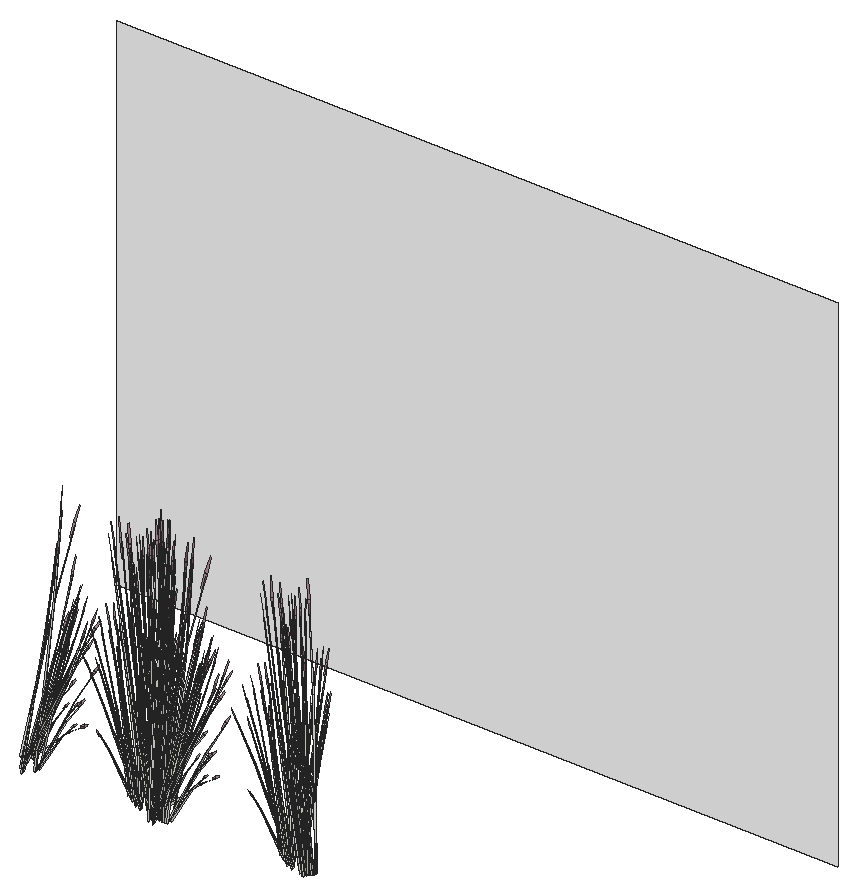
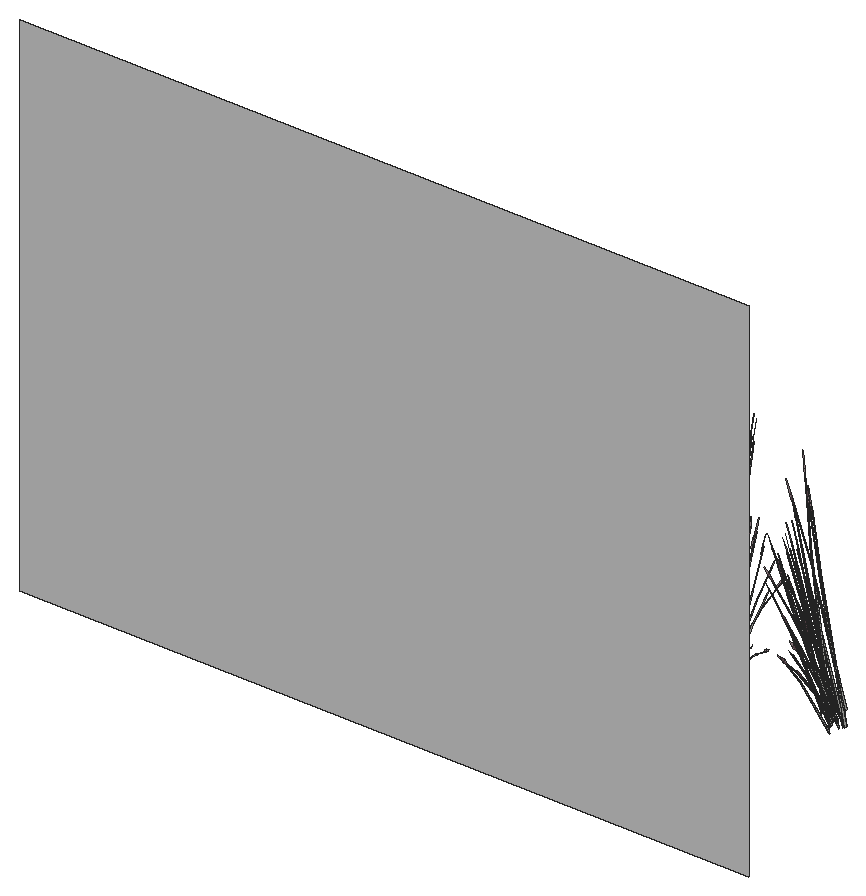
# SketchUp Ruby script. Lengths in inches.
U = 1.inch
M = Sketchup.active_model
def pt(a) = Geom::Point3d.new(a.map { |v| v * U })
def face(e, loops, mat)
  f = e.add_face(loops[0].map { |a| pt(a) })
  loops[1..].each { |l| e.add_face(l.map { |a| pt(a) }).erase! }
  f.material = f.back_material = mat if mat
  f
end
# faces: each face lists its corners as indices into pts; further lists are holes
def faces(e, pts, list, mat = nil) = list.each { |f| face(e, (f[0].is_a?(Array) ? f : [f]).map { |l| l.map { |i| pts[i] } }, mat) }
# xy, xz, yz: faces in a plane at the given z, y or x. An outline is a flat list of corners, or four numbers for a rectangle; further outlines are holes
def ring(l) = l.size == 4 ? [[l[0], l[1]], [l[2], l[1]], [l[2], l[3]], [l[0], l[3]]] : l.each_slice(2).to_a
def flat(e, list, mat, &to3) = list.each { |f| face(e, (f[0].is_a?(Array) ? f : [f]).map { |l| ring(l).map { |u, v| to3.(u, v) } }, mat) }
def xy(e, z, list, mat = nil) = flat(e, list, mat) { |x, y| [x, y, z] }
def xz(e, y, list, mat = nil) = flat(e, list, mat) { |x, z| [x, y, z] }
def yz(e, x, list, mat = nil) = flat(e, list, mat) { |y, z| [x, y, z] }
def lines(e, pts, list) = list.each { |a, b| e.add_line(pt(pts[a]), pt(pts[b])) }
# prism: a flat outline (further loops are holes) pulled along v
def prism(e, loops, v, mat = nil)
  f = face(e, loops, mat); d = Geom::Vector3d.new(v.map { |x| x * U })
  f.pushpull(f.normal.samedirection?(d) ? d.length : -d.length)
end
def box(e, o, s, mat = nil) = prism(e, [[o, [o[0] + s[0], o[1], o[2]], [o[0] + s[0], o[1] + s[1], o[2]], [o[0], o[1] + s[1], o[2]]]], [0, 0, s[2]], mat)
def at(x, y, z, deg = 0) = Geom::Transformation.translation(pt([x, y, z])) * Geom::Transformation.rotation(ORIGIN, Z_AXIS, deg.degrees)
def axes(o, x, y, z) = Geom::Transformation.new([*x, 0, *y, 0, *z, 0, *pt(o).to_a, 1])
def part(name) = M.definitions.add(name)
# library, detail: a bought-in or finely detailed component or shape, given as its bounding box
def library(name, o, s) = part(name).tap { |d| box(d.entities, o, s) }
def detail(e, o, s) = box(e.add_group.entities, o, s)
def put(e, d, t, mat = nil) = e.add_instance(d, t).tap { |i| i.material = mat if mat }
def group(e, t, mat = nil) = e.add_group.tap { |g| g.transformation = t; g.material = mat if mat }.entities
root = M.entities
M.materials.add("LightPink_Translucent").color = [144, 107, 117]
M.materials["LightPink_Translucent"].alpha = 0.75
M.materials.add("M00_Soft_Cloud").color = [255, 255, 255]
c1 = part("blade")
p = [[2.15,0.21,22],[0,0.17,0],[0.09,0.45,0],[2.18,0.31,22],[2.29,0.31,22],[0.38,0.45,0],
  [2.48,0.24,33],[2.49,0.24,33],[2.48,0.22,33]]
faces(c1.entities,p,[[0,1,2,3],[4,5,2,3],[6,3,4,7],[8,0,3,6]])
c2 = part("seeds")
p = [[0.3,-0.1,1.38],[-0.01,-0.03,1.59],[-0.01,-0.03,0.03],[0.14,-0.07,-0.07],[0.29,-0.03,3],[0.15,0.01,3.11]]
faces(c2.entities,p,[[0,1,2,3],[1,0,4,5]],"LightPink_Translucent")
c3 = part("blade with seeds")
put(c3.entities,c1,at(0,0,0))
put(c3.entities,c2,axes([2.4,0.25,30.99],[1.5799,-0.05474,1.17369],[-0.12525,1.92788,0.29478],[-0.07173,-0.02425,1.56792]))
xz(root,72.98,[[57,0,228,120]],"M00_Soft_Cloud")
put(root,c3,axes([113.61,13.07,-3.79],[0.85008,0,0],[0,0.63259,0],[0,0,1.78407]))
put(root,c3,axes([112.17,13.87,-3.33],[-0.76714,0.40567,-0.29095],[-0.51013,-0.57321,-0.50002],[-0.18927,-0.05821,1.59708]))
put(root,c3,axes([148.18,13.87,-3.33],[-0.76714,0.40567,-0.29095],[-0.51013,-0.57321,-0.50002],[-0.18927,-0.05821,1.59708]))
put(root,c3,axes([113.85,11.59,-3.53],[-0.81646,0.16218,0.17642],[-0.20161,-0.60355,0.35086],[0.07282,0.08794,1.60407]))
put(root,c3,axes([83.18,12.86,-2.125],[-0.31515,0.01384,1.71376],[0.20907,-0.5998,0.13857],[0.44912,0.0371,0.73262]))
put(root,c3,axes([114.35,12.86,-2.125],[-0.31515,0.01384,1.71376],[0.20907,-0.5998,0.13857],[0.44912,0.0371,0.73262]))
put(root,c3,axes([83.59,11.56,-3.97],[0.17848,0.53243,-0.30978],[-0.70886,0.15119,0.30978],[0.1429,0.0614,1.38974]))
put(root,c3,axes([114.76,11.56,-3.97],[0.17848,0.53243,-0.30978],[-0.70886,0.15119,0.30978],[0.1429,0.0614,1.38974]))
put(root,c3,axes([84.81,13.6875,-1.27],[0.27906,0.41663,0.0643],[-0.50888,0.20393,0.50621],[0.22432,-0.04024,0.77189]))
put(root,c3,axes([115.98,13.6875,-1.27],[0.27906,0.41663,0.0643],[-0.50888,0.20393,0.50621],[0.22432,-0.04024,0.77189]))
put(root,c3,axes([113.34,12.75,-3.62],[-0.96033,-0.12874,0.49198],[0.19544,-0.7271,0.19306],[0.14034,0.07021,1.70813]))
put(root,c3,axes([84.75,13.54,-1.27],[-0.21466,0.55714,0.48003],[-0.70573,-0.19051,0.3958],[0.27753,-0.03348,0.9933]))
put(root,c3,axes([115.93,13.54,-1.27],[-0.21466,0.55714,0.48003],[-0.70573,-0.19051,0.3958],[0.27753,-0.03348,0.9933]))
put(root,c3,axes([112.57,14.55,-3.8],[-0.24791,-0.5268,0],[0.70791,-0.18448,0],[0,0,1.54371]))
put(root,c3,axes([112.1,14.05,-3.38],[-0.14658,0.54532,0.1448],[-0.71613,-0.09466,-0.41347],[-0.13033,-0.05599,1.26744]))
put(root,c3,axes([148.11,14.05,-3.38],[-0.14658,0.54532,0.1448],[-0.71613,-0.09466,-0.41347],[-0.13033,-0.05599,1.26744]))
put(root,c3,axes([109.32,12.63,-0.95],[0.63144,0.17046,0.35414],[-0.18417,0.49731,-0.4572],[-0.25423,0.0456,0.87481]))
put(root,c3,axes([145.33,12.63,-0.95],[0.63144,0.17046,0.35414],[-0.18417,0.49731,-0.4572],[-0.25423,0.0456,0.87481]))
put(root,c3,axes([113.5,14.47,-3.82],[0.79769,-0.20732,-0.19198],[0.2803,0.59721,0.00008],[0.08805,-0.02292,1.73897]))
put(root,c3,axes([113.77,14.72,-3.53],[0.21949,-0.60727,0.17642],[0.8032,0.17185,0.35086],[-0.13875,0.00296,1.60407]))
put(root,c3,axes([149.79,14.72,-3.53],[0.21949,-0.60727,0.17642],[0.8032,0.17185,0.35086],[-0.13875,0.00296,1.60407]))
put(root,c3,axes([113.59,13.34,-3.79],[0.53038,0.39469,0],[-0.53038,0.39469,0],[0,0,1.69266]))
put(root,c3,axes([110.58,12.6,-2.66],[0.21597,-0.08839,1.77064],[0.07448,0.61717,0.13857],[-0.4678,0.08189,0.63284]))
put(root,c3,axes([146.59,12.6,-2.66],[0.21597,-0.08839,1.77064],[0.07448,0.61717,0.13857],[-0.4678,0.08189,0.63284]))
put(root,c3,axes([115.03,13.17,-3.53],[-0.59697,-0.44509,0.17642],[0.60159,-0.4317,0.35086],[-0.06593,0.0909,1.60407]))
put(root,c3,axes([82.75,12.5,-3.94],[0.79037,0.10018,-0.62353],[-0.16679,0.61794,-0.16365],[0.23587,0.07488,1.37633]))
put(root,c3,axes([113.92,12.5,-3.94],[0.79037,0.10018,-0.62353],[-0.16679,0.61794,-0.16365],[0.23587,0.07488,1.37633]))
put(root,c3,axes([86.24,13.58,-3.23],[-0.46945,0.10088,1.1486],[0.22097,-0.4169,0.84392],[0.24904,0.02853,0.25299]))
put(root,c3,axes([117.41,13.58,-3.23],[-0.46945,0.10088,1.1486],[0.22097,-0.4169,0.84392],[0.24904,0.02853,0.25299]))
put(root,c3,axes([112.39,14.78,-3.8],[-0.76598,-0.27433,0],[0.36864,-0.57001,0],[0,0,1.62707]))
put(root,c3,axes([148.41,14.78,-3.8],[-0.76598,-0.27433,0],[0.36864,-0.57001,0],[0,0,1.62707]))
put(root,c3,axes([113.03,14.05,-3.54],[-0.74193,-0.49181,-0.25192],[0.6243,-0.55226,0.5513],[-0.19979,0.05753,1.68216]))
put(root,c3,axes([149.04,14.05,-3.54],[-0.74193,-0.49181,-0.25192],[0.6243,-0.55226,0.5513],[-0.19979,0.05753,1.68216]))
put(root,c3,axes([111.08,15,-3.52],[0.7111,0.30552,0.49651],[-0.42504,0.54784,0],[-0.16196,-0.06958,1.57504]))
put(root,c3,axes([147.09,15,-3.52],[0.7111,0.30552,0.49651],[-0.42504,0.54784,0],[-0.16196,-0.06958,1.57504]))
put(root,c3,axes([113.58,12.88,-3.28],[0.36864,-0.55059,0.44739],[0.76598,0.26498,-0.21531],[0,0.12692,1.43643]))
put(root,c3,axes([86.02,15.34,-1.29],[-0.0687,-0.05349,1.77383],[0.15029,-0.57341,-0.16761],[0.27062,-0.03664,0.31391]))
put(root,c3,axes([117.2,15.34,-1.29],[-0.0687,-0.05349,1.77383],[0.15029,-0.57341,-0.16761],[0.27062,-0.03664,0.31391]))
put(root,c3,axes([108.25,13.02,-1.28],[-0.12407,0.07933,1.74944],[0.01055,0.57963,-0.27667],[-0.2844,0.07538,0.14031]))
put(root,c3,axes([144.27,13.02,-1.28],[-0.12407,0.07933,1.74944],[0.01055,0.57963,-0.27667],[-0.2844,0.07538,0.14031]))
put(root,c3,axes([113.44,13.2,-3.71],[0,0.70667,-0.05637],[-0.95008,0,0],[0,0.02221,1.79368]))
put(root,c3,axes([109.09,12.94,-1.32],[-0.20584,0.55581,-0.51099],[-0.70573,-0.19051,-0.3958],[-0.28414,0.05097,0.97773]))
put(root,c3,axes([145.1,12.94,-1.32],[-0.20584,0.55581,-0.51099],[-0.70573,-0.19051,-0.3958],[-0.28414,0.05097,0.97773]))
put(root,c3,axes([109.05,12.46,-0.97],[0.38229,0.5533,-0.1216],[-0.6785,0.2719,-0.67495],[-0.28593,0.073,1.02557]))
put(root,c3,axes([145.07,12.46,-0.97],[0.38229,0.5533,-0.1216],[-0.6785,0.2719,-0.67495],[-0.28593,0.073,1.02557]))
put(root,c3,axes([82.34,12.7,-3.79],[0.45644,0.51287,-0.44739],[-0.69137,0.36116,0.21531],[0.14771,0.06346,1.43643]))
put(root,c3,axes([113.51,12.7,-3.79],[0.45644,0.51287,-0.44739],[-0.69137,0.36116,0.21531],[0.14771,0.06346,1.43643]))
put(root,c3,axes([85.42,14.87,-2.07],[-0.14542,-0.51365,-0.03492],[0.68734,-0.11809,-0.15832],[0.14353,0.03256,0.52218]))
put(root,c3,axes([116.6,14.87,-2.07],[-0.14542,-0.51365,-0.03492],[0.68734,-0.11809,-0.15832],[0.14353,0.03256,0.52218]))
put(root,c3,axes([110.67,15.32,-3.625],[-0.47504,0.61229,0],[-0.79476,-0.34146,-0.51607],[-0.18101,-0.07777,1.63711]))
put(root,c3,axes([146.68,15.32,-3.625],[-0.47504,0.61229,0],[-0.79476,-0.34146,-0.51607],[-0.18101,-0.07777,1.63711]))
put(root,c3,axes([83.64,14.85,-0.97],[0.04068,-0.62141,-0.1216],[0.77029,0.01698,-0.67495],[0.29667,0.04317,1.02557]))
put(root,c3,axes([114.82,14.85,-0.97],[0.04068,-0.62141,-0.1216],[0.77029,0.01698,-0.67495],[0.29667,0.04317,1.02557]))
put(root,c3,axes([115.52,13.19,-3.52],[0,-0.61104,0.49651],[0.85008,0,0],[0,0.13917,1.57504]))
put(root,c3,axes([113.39,13.65,-3.28],[0.82508,-0.03772,0.44739],[0.07462,0.62614,-0.21531],[-0.14771,0.06346,1.43643]))
put(root,c3,axes([149.4,13.65,-3.28],[0.82508,-0.03772,0.44739],[0.07462,0.62614,-0.21531],[-0.14771,0.06346,1.43643]))
put(root,c3,axes([113.9,13.01,-3.38],[0.70791,-0.1782,0.1448],[0.24791,0.50885,-0.41347],[0,0.11199,1.26744]))
put(root,c3,axes([83.52,14.61,-0.95],[-0.43232,-0.38257,0.35414],[0.49364,-0.36215,-0.4572],[0.25081,0.0551,0.87481]))
put(root,c3,axes([114.7,14.61,-0.95],[-0.43232,-0.38257,0.35414],[0.49364,-0.36215,-0.4572],[0.25081,0.0551,0.87481]))
put(root,c3,axes([112.65,13.95,-3.79],[-0.82508,0.03772,-0.44739],[-0.07462,-0.62614,0.21531],[-0.14771,0.06346,1.43643]))
put(root,c3,axes([148.67,13.95,-3.79],[-0.82508,0.03772,-0.44739],[-0.07462,-0.62614,0.21531],[-0.14771,0.06346,1.43643]))
put(root,c3,axes([85.36,14.25,-3.41],[-0.18299,-0.15028,1.43002],[0.23809,-0.49714,-0.30754],[0.37023,0.06735,0.61141]))
put(root,c3,axes([116.53,14.25,-3.41],[-0.18299,-0.15028,1.43002],[0.23809,-0.49714,-0.30754],[0.37023,0.06735,0.61141]))
put(root,c3,axes([113.26,14.8,-3.8],[0.76598,0.27433,0],[-0.36864,0.57001,0],[0,0,1.74954]))
put(root,c3,axes([84.3125,14.48,-1.28],[0.16299,-0.01033,1.74944],[0.44707,-0.47471,-0.27667],[0.28992,0.06266,0.14031]))
put(root,c3,axes([115.49,14.48,-1.28],[0.16299,-0.01033,1.74944],[0.44707,-0.47471,-0.27667],[0.28992,0.06266,0.14031]))
put(root,c3,axes([113.57,15.4,-3.81],[-0.46912,-0.61443,-0.05142],[0.79476,-0.34146,0.51607],[-0.19584,0.0585,1.6363]))
put(root,c3,axes([149.58,15.4,-3.81],[-0.46912,-0.61443,-0.05142],[0.79476,-0.34146,0.51607],[-0.19584,0.0585,1.6363]))
put(root,c3,axes([113.4,13.92,-3.38],[0.56134,0.36712,0.1448],[-0.46823,0.41419,-0.41347],[-0.13033,0.05599,1.26744]))
put(root,c3,axes([149.42,13.92,-3.38],[0.56134,0.36712,0.1448],[-0.46823,0.41419,-0.41347],[-0.13033,0.05599,1.26744]))
put(root,c3,axes([108.97,14.01,-1.27],[-0.18844,-0.56237,0.48003],[0.73919,-0.0976,0.3958],[-0.21785,0.13226,0.9933]))
put(root,c3,axes([144.98,14.01,-1.27],[-0.18844,-0.56237,0.48003],[0.73919,-0.0976,0.3958],[-0.21785,0.13226,0.9933]))
put(root,c3,axes([108.82,13.9,-1.27],[-0.52161,-0.25698,0.0643],[0.30368,-0.36595,0.50621],[-0.16723,0.11831,0.77189]))
put(root,c3,axes([144.84,13.9,-1.27],[-0.52161,-0.25698,0.0643],[0.30368,-0.36595,0.50621],[-0.16723,0.11831,0.77189]))
put(root,c3,axes([109.0625,13.23,-2.125],[0.26363,-0.12925,1.71376],[0.22195,0.59723,0.13857],[-0.41388,0.13498,0.73262]))
put(root,c3,axes([145.08,13.23,-2.125],[0.26363,-0.12925,1.71376],[0.22195,0.59723,0.13857],[-0.41388,0.13498,0.73262]))
put(root,c3,axes([83.68,14.55,-1.02],[0.75952,0.01471,-0.71045],[-0.05101,0.61953,0.08574],[0.32177,0.06538,1.00501]))
put(root,c3,axes([114.86,14.55,-1.02],[0.75952,0.01471,-0.71045],[-0.05101,0.61953,0.08574],[0.32177,0.06538,1.00501]))
put(root,c3,axes([114,15.05,-3.52],[0.7111,-0.30552,0.49651],[0.42504,0.54784,0],[-0.16196,0.06958,1.57504]))
put(root,c3,axes([112.99,14.57,-3.71],[0.33034,0.70197,-0.06012],[-0.94388,0.24598,0],[0.01154,0.02451,1.72173]))
put(root,c3,axes([113.35,15.32,-3.97],[-0.70886,-0.15119,-0.30978],[0.17848,-0.53243,0.30978],[-0.1429,0.0614,1.38974]))
put(root,c3,axes([149.37,15.32,-3.97],[-0.70886,-0.15119,-0.30978],[0.17848,-0.53243,0.30978],[-0.1429,0.0614,1.38974]))
put(root,c3,axes([108.24,14.24,-3.41],[0.26405,0.05016,1.43002],[0.17019,0.51235,-0.30754],[-0.35868,0.0959,0.61141]))
put(root,c3,axes([144.25,14.24,-3.41],[0.26405,0.05016,1.43002],[0.17019,0.51235,-0.30754],[-0.35868,0.0959,0.61141]))
put(root,c3,axes([109.42,13.83,-0.95],[0.66138,-0.08733,0.35414],[0.17464,0.49921,-0.4572],[-0.18953,0.13408,0.87481]))
put(root,c3,axes([145.4375,13.83,-0.95],[0.66138,-0.08733,0.35414],[0.17464,0.49921,-0.4572],[-0.18953,0.13408,0.87481]))
put(root,c3,axes([84.92,13.29,-3.625],[0.95008,0,0],[0,0.68292,-0.51607],[0,0.15554,1.63711]))
put(root,c3,axes([116.1,13.29,-3.625],[0.95008,0,0],[0,0.68292,-0.51607],[0,0.15554,1.63711]))
put(root,c3,axes([106.875,13.6,-1.29],[0.09697,0.01639,1.77383],[0.29997,0.53988,-0.16761],[-0.1985,0.1417,0.31391]))
put(root,c3,axes([142.89,13.6,-1.29],[0.09697,0.01639,1.77383],[0.29997,0.53988,-0.16761],[-0.1985,0.1417,0.31391]))
put(root,c3,axes([115.72,13.64,-3.8],[-0.94962,-0.00489,-0.04976],[0,-0.68292,0.49943],[-0.02984,0.15546,1.58352]))
put(root,c3,axes([113.66,13.05,-3.33],[0.85568,0.29155,-0.29095],[-0.41201,0.61537,-0.50002],[0.02689,0.15109,1.59708]))
put(root,c3,axes([107.69,15.32,-3.23],[0.31665,-0.27694,1.1486],[0.12495,0.43841,0.84392],[-0.22883,0.0785,0.25299]))
put(root,c3,axes([143.7,15.32,-3.23],[0.31665,-0.27694,1.1486],[0.12495,0.43841,0.84392],[-0.22883,0.0785,0.25299]))
put(root,c3,axes([84.14,14.81,-1.47],[0.43232,0.38257,-0.35414],[-0.49364,0.36215,0.4572],[0.25081,0.0551,0.87481]))
put(root,c3,axes([115.3125,14.81,-1.47],[0.43232,0.38257,-0.35414],[-0.49364,0.36215,0.4572],[0.25081,0.0551,0.87481]))
put(root,c3,axes([115.52,13.74,-3.97],[-0.53038,0.38124,-0.30978],[-0.53038,-0.38124,0.30978],[0,0.1228,1.38974]))
put(root,c3,axes([113.23,13.78,-3.33],[0.08854,0.69723,-0.29095],[-0.92215,0.04216,-0.50002],[-0.16238,0.09287,1.59708]))
put(root,c3,axes([149.25,13.78,-3.33],[0.08854,0.69723,-0.29095],[-0.92215,0.04216,-0.50002],[-0.16238,0.09287,1.59708]))
put(root,c3,axes([83.91,14.95,-1.27],[-0.03826,0.46465,0.0643],[-0.57772,-0.01274,0.50621],[0.2213,0.04862,0.77189]))
put(root,c3,axes([115.09,14.95,-1.27],[-0.03826,0.46465,0.0643],[-0.57772,-0.01274,0.50621],[0.2213,0.04862,0.77189]))
put(root,c3,axes([113.57,13.51,-3.79],[-0.36864,0.55059,-0.44739],[-0.76598,-0.26498,0.21531],[0,0.12692,1.43643]))
put(root,c3,axes([108.88,14.12,-1.47],[-0.66138,0.08733,-0.35414],[-0.17464,-0.49921,0.4572],[-0.18953,0.13408,0.87481]))
put(root,c3,axes([144.9,14.12,-1.47],[-0.66138,0.08733,-0.35414],[-0.17464,-0.49921,0.4572],[-0.18953,0.13408,0.87481]))
put(root,c3,axes([83.97,14.81,-1.27],[-0.56024,0.40262,0.48003],[-0.48318,-0.42758,0.3958],[0.26285,0.07427,0.9933]))
put(root,c3,axes([115.14,14.81,-1.27],[-0.56024,0.40262,0.48003],[-0.48318,-0.42758,0.3958],[0.26285,0.07427,0.9933]))
put(root,c3,axes([107.92,15.24,-0.35],[0.67048,0.16311,-0.06488],[-0.20625,0.50201,-0.29416],[-0.10966,0.07622,0.97024]))
put(root,c3,axes([143.9375,15.24,-0.35],[0.67048,0.16311,-0.06488],[-0.20625,0.50201,-0.29416],[-0.10966,0.07622,0.97024]))
put(root,c3,axes([112.68,14.3125,-3.94],[-0.51177,0.45928,-0.62353],[-0.63575,-0.41646,-0.16365],[-0.20507,0.11457,1.37633]))
put(root,c3,axes([148.69,14.3125,-3.94],[-0.51177,0.45928,-0.62353],[-0.63575,-0.41646,-0.16365],[-0.20507,0.11457,1.37633]))
put(root,c3,axes([113.36,15.27,-0.95],[-0.11735,-0.49217,0.35414],[0.67083,-0.12996,-0.4572],[0.18018,0.14104,0.87481]))
put(root,c3,axes([113.59,15.09,-3.67],[0.95122,0.19861,0.30756],[-0.23797,0.7099,-0.36492],[-0.15744,0.08885,1.64885]))
put(root,c3,axes([113.52,15.57,-3.98],[-0.7111,0.30552,-0.49651],[-0.42504,-0.54784,0],[-0.16196,0.06958,1.57504]))
put(root,c3,axes([149.54,15.57,-3.98],[-0.7111,0.30552,-0.49651],[-0.42504,-0.54784,0],[-0.16196,0.06958,1.57504]))
put(root,c3,axes([115.88,13.76,-3.98],[0,0.61104,-0.49651],[-0.85008,0,0],[0,0.13917,1.57504]))
put(root,c3,axes([82.58,13.83,-2.125],[-0.28223,-0.10528,1.71376],[0.58406,-0.44165,0.13857],[0.36402,0.19924,0.73262]))
put(root,c3,axes([113.76,13.83,-2.125],[-0.28223,-0.10528,1.71376],[0.58406,-0.44165,0.13857],[0.36402,0.19924,0.73262]))
put(root,c3,axes([82.64,12.44,-1.53],[-0.65655,-0.31748,1.38283],[0.69326,-0.49431,0.59665],[0.21183,0.29789,1.33663]))
put(root,c3,axes([113.8125,12.44,-1.53],[-0.65655,-0.31748,1.38283],[0.69326,-0.49431,0.59665],[0.21183,0.29789,1.33663]))
put(root,c3,axes([109.08,13.78,-0.97],[0.70283,0.33692,-0.1216],[-0.40491,0.48793,-0.67495],[-0.19857,0.16961,1.02557]))
put(root,c3,axes([145.09,13.78,-0.97],[0.70283,0.33692,-0.1216],[-0.40491,0.48793,-0.67495],[-0.19857,0.16961,1.02557]))
put(root,c3,axes([83.63,15.02,-3.23],[-0.4278,-0.1757,1.1486],[0.5524,-0.17852,0.84392],[0.14899,0.15122,0.25299]))
put(root,c3,axes([114.8,15.02,-3.23],[-0.4278,-0.1757,1.1486],[0.5524,-0.17852,0.84392],[0.14899,0.15122,0.25299]))
put(root,c3,axes([82.125,15.53,-0.97],[0.45276,-0.52302,-0.1216],[0.65568,0.30132,-0.67495],[0.22792,0.14777,1.02557]))
put(root,c3,axes([113.3,15.53,-0.97],[0.45276,-0.52302,-0.1216],[0.65568,0.30132,-0.67495],[0.22792,0.14777,1.02557]))
put(root,c3,axes([110.03,13.63,-2.125],[0.18977,-0.18775,1.71376],[0.47917,0.50677,0.13857],[-0.32866,0.23079,0.73262]))
put(root,c3,axes([146.04,13.63,-2.125],[0.18977,-0.18775,1.71376],[0.47917,0.50677,0.13857],[-0.32866,0.23079,0.73262]))
put(root,c3,axes([109.43,14.18,-1.32],[0.19519,0.55794,-0.51099],[-0.73919,0.0976,-0.3958],[-0.21183,0.14986,0.97773]))
put(root,c3,axes([145.44,14.18,-1.32],[0.19519,0.55794,-0.51099],[-0.73919,0.0976,-0.3958],[-0.21183,0.14986,0.97773]))
put(root,c3,axes([110.32,14.82,-0.95],[0.5141,-0.32171,0.35414],[0.48666,0.36734,-0.4572],[-0.07405,0.18664,0.87481]))
put(root,c3,axes([146.33,14.82,-0.95],[0.5141,-0.32171,0.35414],[0.48666,0.36734,-0.4572],[-0.07405,0.18664,0.87481]))
put(root,c3,axes([114.17,15.47,-3.625],[0.47504,0.61229,0],[-0.79476,0.34146,-0.51607],[-0.18101,0.07777,1.63711]))
put(root,c3,axes([150.18,15.47,-3.625],[0.47504,0.61229,0],[-0.79476,0.34146,-0.51607],[-0.18101,0.07777,1.63711]))
put(root,c3,axes([81.53,15.96,-1.29],[0.00225,-0.07398,1.77383],[0.65113,-0.32638,-0.16761],[0.22617,0.1165,0.31391]))
put(root,c3,axes([112.71,15.96,-1.29],[0.00225,-0.07398,1.77383],[0.65113,-0.32638,-0.16761],[0.22617,0.1165,0.31391]))
put(root,c3,axes([83.75,15.68,-4.51],[0.05536,-0.08822,1.76342],[0.69692,-0.25981,-0.26939],[0.21129,0.13447,0.30037]))
put(root,c3,axes([114.92,15.68,-4.51],[0.05536,-0.08822,1.76342],[0.69692,-0.25981,-0.26939],[0.21129,0.13447,0.30037]))
put(root,c3,axes([113.76,13.05,-3.16],[-0.02076,-0.57531,1.41272],[0.93937,0.14913,0.59816],[-0.22217,0.31481,1.3335]))
put(root,c3,axes([149.78,13.05,-3.16],[-0.02076,-0.57531,1.41272],[0.93937,0.14913,0.59816],[-0.22217,0.31481,1.3335]))
put(root,c3,axes([114,13.67,-3.91],[0.2786,0.55945,-0.69212],[-0.80253,0.20149,-0.18165],[0.03079,0.18945,1.52773]))
put(root,c3,axes([109.85,15.11,-1.27],[-0.62439,-0.02847,0.0643],[0.01712,-0.42991,0.50621],[-0.06534,0.16468,0.77189]))
put(root,c3,axes([145.86,15.11,-1.27],[-0.62439,-0.02847,0.0643],[0.01712,-0.42991,0.50621],[-0.06534,0.16468,0.77189]))
put(root,c3,axes([108.52,15.6,-4.51],[0.10192,0.06105,1.76342],[0.17281,0.56562,-0.26939],[-0.22588,0.12062,0.30037]))
put(root,c3,axes([144.54,15.6,-4.51],[0.10192,0.06105,1.76342],[0.17281,0.56562,-0.26939],[-0.22588,0.12062,0.30037]))
put(root,c3,axes([110.05,15.15,-1.27],[-0.54105,-0.41691,0.48003],[0.57458,-0.35956,0.3958],[-0.0998,0.1956,0.9933]))
put(root,c3,axes([146.0625,15.15,-1.27],[-0.54105,-0.41691,0.48003],[0.57458,-0.35956,0.3958],[-0.0998,0.1956,0.9933]))
put(root,c3,axes([82.66,15.27,-1.32],[0.74975,-0.14525,-0.51099],[0.13115,0.55007,-0.3958],[0.20138,0.15763,0.97773]))
put(root,c3,axes([113.84,15.27,-1.32],[0.74975,-0.14525,-0.51099],[0.13115,0.55007,-0.3958],[0.20138,0.15763,0.97773]))
put(root,c3,axes([111.76,15.35,-0.95],[0.22906,-0.4699,0.35414],[0.66828,0.13705,-0.4572],[0.06128,0.18919,0.87481]))
put(root,c3,axes([83.7,15.82,-3.33],[-0.48723,-0.01916,1.0506],[0.32177,-0.40701,0.58006],[0.19248,0.1446,0.8241]))
put(root,c3,axes([114.87,15.82,-3.33],[-0.48723,-0.01916,1.0506],[0.32177,-0.40701,0.58006],[0.19248,0.1446,0.8241]))
put(root,c3,axes([113.47,15.72,-1.27],[-0.34533,0.38816,0.0643],[-0.49176,-0.22599,0.50621],[0.15898,0.12445,0.77189]))
put(root,c3,axes([112.66,17.03,-0.35],[0.52505,-0.35054,-0.06488],[0.48109,0.38392,-0.29416],[0.03387,0.10878,0.97024]))
put(root,c3,axes([113.61,15.61,-1.27],[-0.75571,0.14023,0.48003],[-0.13115,-0.55007,0.3958],[0.17773,0.16212,0.9933]))
put(root,c3,axes([109.88,14.09,-2.125],[0.14147,-0.21002,1.71376],[0.59349,0.43464,0.13857],[-0.26773,0.27089,0.73262]))
put(root,c3,axes([145.9,14.09,-2.125],[0.14147,-0.21002,1.71376],[0.59349,0.43464,0.13857],[-0.26773,0.27089,0.73262]))
put(root,c3,axes([82.1,14.84,-3.41],[0.01341,-0.20255,1.43002],[0.64074,-0.22625,-0.30754],[0.1978,0.24243,0.61141]))
put(root,c3,axes([113.28,14.84,-3.41],[0.01341,-0.20255,1.43002],[0.64074,-0.22625,-0.30754],[0.1978,0.24243,0.61141]))
put(root,c3,axes([111.55,15.77,-1.27],[-0.55987,0.20767,0.0643],[-0.27403,-0.37869,0.50621],[0.05407,0.16693,0.77189]))
put(root,c3,axes([147.5625,15.77,-1.27],[-0.55987,0.20767,0.0643],[-0.27403,-0.37869,0.50621],[0.05407,0.16693,0.77189]))
put(root,c3,axes([110.05,15.28,-1.47],[-0.5141,0.32171,-0.35414],[-0.48666,-0.36734,0.4572],[-0.07405,0.18664,0.87481]))
put(root,c3,axes([146.0625,15.28,-1.47],[-0.5141,0.32171,-0.35414],[-0.48666,-0.36734,0.4572],[-0.07405,0.18664,0.87481]))
put(root,c3,axes([108.28,15.18,-1.28],[-0.01889,0.12092,1.74944],[0.53598,0.42065,-0.27667],[-0.14032,0.19892,0.14031]))
put(root,c3,axes([144.29,15.18,-1.28],[-0.01889,0.12092,1.74944],[0.53598,0.42065,-0.27667],[-0.14032,0.19892,0.14031]))
put(root,c3,axes([109.99,14.91,-0.6],[0.83505,0.03027,-0.13498],[-0.02282,0.57322,-0.74919],[-0.05801,0.22077,1.13838]))
put(root,c3,axes([146,14.91,-0.6],[0.83505,0.03027,-0.13498],[-0.02282,0.57322,-0.74919],[-0.05801,0.22077,1.13838]))
put(root,c3,axes([111.53,15.55,-0.97],[0.74352,-0.28449,-0.1216],[0.36538,0.50492,-0.67495],[0.0981,0.21277,1.02557]))
put(root,c3,axes([111.75,15.73,-0.9375],[-0.74868,-0.15974,0.53283],[0.25601,-0.52518,0.43934],[0.04499,0.20653,1.10256]))
put(root,c3,axes([147.76,15.73,-0.9375],[-0.74868,-0.15974,0.53283],[0.25601,-0.52518,0.43934],[0.04499,0.20653,1.10256]))
put(root,c3,axes([110.375,16.53,-3.23],[-0.01966,-0.36332,1.1486],[0.49135,0.25914,0.84392],[-0.09663,0.17317,0.25299]))
put(root,c3,axes([146.39,16.53,-3.23],[-0.01966,-0.36332,1.1486],[0.49135,0.25914,0.84392],[-0.09663,0.17317,0.25299]))
put(root,c3,axes([111.67,15.66,-4.51],[0.12297,-0.03325,1.76342],[0.73967,0.18301,-0.26939],[0.02163,0.20626,0.30037]))
put(root,c3,axes([110.56,15.125,-1],[0.54391,0.41056,-0.5672],[-0.57458,0.35956,-0.43934],[-0.08276,0.2086,1.08528]))
put(root,c3,axes([146.57,15.125,-1],[0.54391,0.41056,-0.5672],[-0.57458,0.35956,-0.43934],[-0.08276,0.2086,1.08528]))
put(root,c3,axes([109.97,15.74,-3.18],[0.69024,-0.1082,0.06507],[0.15868,0.43593,-0.86304],[-0.04376,0.22067,0.7736]))
put(root,c3,axes([145.98,15.74,-3.18],[0.69024,-0.1082,0.06507],[0.15868,0.43593,-0.86304],[-0.04376,0.22067,0.7736]))
put(root,c3,axes([112.17,15.52,-1.32],[0.7469,0.15318,-0.51099],[-0.25601,0.52518,-0.3958],[0.06849,0.21144,0.97773]))
put(root,c3,axes([112.6,14.4375,-2.125],[-0.17368,-0.19618,1.71376],[0.80256,-0.16516,0.13857],[0.18139,0.30799,0.73262]))
put(root,c3,axes([111.83,15.84,-1.47],[-0.22906,0.4699,-0.35414],[-0.66828,-0.13705,0.4572],[0.06128,0.18919,0.87481]))
put(root,c3,axes([110.39,14.9375,-0.66],[-0.01977,0.56521,-0.7886],[-0.83252,-0.03796,0.09517],[-0.08786,0.23945,1.11556]))
put(root,c3,axes([146.4,14.9375,-0.66],[-0.01977,0.56521,-0.7886],[-0.83252,-0.03796,0.09517],[-0.08786,0.23945,1.11556]))
put(root,c3,axes([108.21,16.42,-1.29],[0.0862,-0.03689,1.77383],[0.71245,0.24539,-0.16761],[-0.01674,0.20431,0.31391]))
put(root,c3,axes([144.23,16.42,-1.29],[0.0862,-0.03689,1.77383],[0.71245,0.24539,-0.16761],[-0.01674,0.20431,0.31391]))
put(root,c3,axes([111.18,14.54,-2.125],[-0.0186,-0.23452,1.71376],[0.80601,0.15558,0.13857],[-0.04985,0.33422,0.73262]))
put(root,c3,axes([147.19,14.54,-2.125],[-0.0186,-0.23452,1.71376],[0.80601,0.15558,0.13857],[-0.04985,0.33422,0.73262]))
put(root,c3,axes([111.9,15.42,-1.02],[0.36264,0.49684,-0.71045],[-0.74649,0.27689,0.08574],[0.0848,0.24006,1.00501]))
put(root,c3,axes([109.8,16.2,-3.41],[0.23977,-0.09639,1.43002],[0.59198,0.29065,-0.30754],[-0.1762,0.25149,0.61141]))
put(root,c3,axes([145.82,16.2,-3.41],[0.23977,-0.09639,1.43002],[0.59198,0.29065,-0.30754],[-0.1762,0.25149,0.61141]))
put(root,c3,axes([111.36,16.68,-1.28],[0.09631,0.0984,1.74944],[0.77725,0.03866,-0.27667],[0.07816,0.217,0.14031]))
put(root,c3,axes([110.11,15.73,-2.64],[0.01669,-0.31544,1.54345],[0.75083,0.16661,0.21329],[-0.06506,0.33618,0.72882]))
put(root,c3,axes([146.125,15.73,-2.64],[0.01669,-0.31544,1.54345],[0.75083,0.16661,0.21329],[-0.06506,0.33618,0.72882]))
